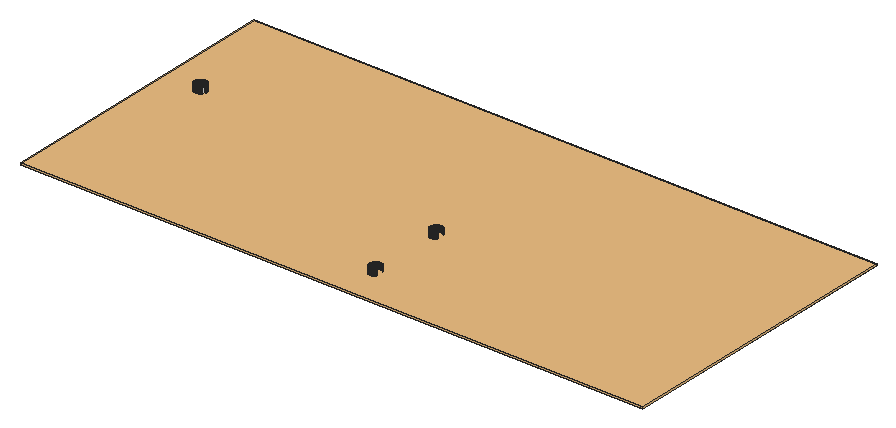
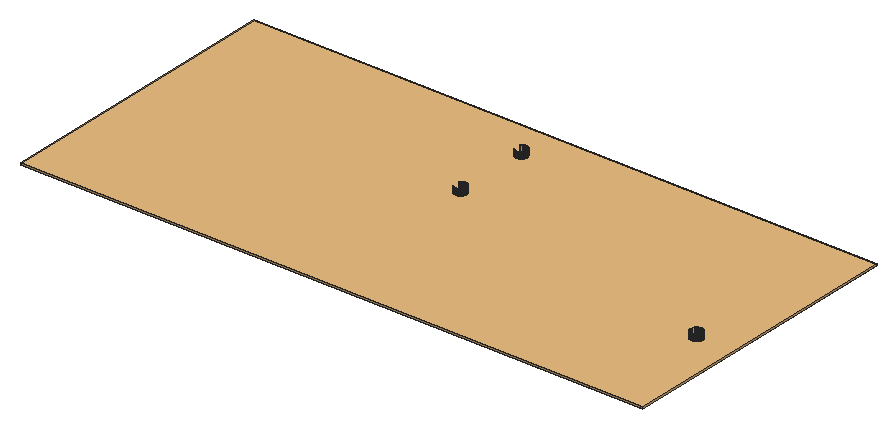
# SketchUp Ruby script. Lengths in inches.
U = 1.inch
M = Sketchup.active_model
def pt(a) = Geom::Point3d.new(a.map { |v| v * U })
def face(e, loops, mat)
  f = e.add_face(loops[0].map { |a| pt(a) })
  loops[1..].each { |l| e.add_face(l.map { |a| pt(a) }).erase! }
  f.material = f.back_material = mat if mat
  f
end
# faces: each face lists its corners as indices into pts; further lists are holes
def faces(e, pts, list, mat = nil) = list.each { |f| face(e, (f[0].is_a?(Array) ? f : [f]).map { |l| l.map { |i| pts[i] } }, mat) }
# xy, xz, yz: faces in a plane at the given z, y or x. An outline is a flat list of corners, or four numbers for a rectangle; further outlines are holes
def ring(l) = l.size == 4 ? [[l[0], l[1]], [l[2], l[1]], [l[2], l[3]], [l[0], l[3]]] : l.each_slice(2).to_a
def flat(e, list, mat, &to3) = list.each { |f| face(e, (f[0].is_a?(Array) ? f : [f]).map { |l| ring(l).map { |u, v| to3.(u, v) } }, mat) }
def xy(e, z, list, mat = nil) = flat(e, list, mat) { |x, y| [x, y, z] }
def xz(e, y, list, mat = nil) = flat(e, list, mat) { |x, z| [x, y, z] }
def yz(e, x, list, mat = nil) = flat(e, list, mat) { |y, z| [x, y, z] }
def lines(e, pts, list) = list.each { |a, b| e.add_line(pt(pts[a]), pt(pts[b])) }
# prism: a flat outline (further loops are holes) pulled along v
def prism(e, loops, v, mat = nil)
  f = face(e, loops, mat); d = Geom::Vector3d.new(v.map { |x| x * U })
  f.pushpull(f.normal.samedirection?(d) ? d.length : -d.length)
end
def box(e, o, s, mat = nil) = prism(e, [[o, [o[0] + s[0], o[1], o[2]], [o[0] + s[0], o[1] + s[1], o[2]], [o[0], o[1] + s[1], o[2]]]], [0, 0, s[2]], mat)
def at(x, y, z, deg = 0) = Geom::Transformation.translation(pt([x, y, z])) * Geom::Transformation.rotation(ORIGIN, Z_AXIS, deg.degrees)
def axes(o, x, y, z) = Geom::Transformation.new([*x, 0, *y, 0, *z, 0, *pt(o).to_a, 1])
def part(name) = M.definitions.add(name)
# library, detail: a bought-in or finely detailed component or shape, given as its bounding box
def library(name, o, s) = part(name).tap { |d| box(d.entities, o, s) }
def detail(e, o, s) = box(e.add_group.entities, o, s)
def put(e, d, t, mat = nil) = e.add_instance(d, t).tap { |i| i.material = mat if mat }
def group(e, t, mat = nil) = e.add_group.tap { |g| g.transformation = t; g.material = mat if mat }.entities
root = M.entities
M.materials.add("False Ceiling Light").color = [251, 213, 131]
c1 = library("Group\#31",[0,0,0],[264,124,0.5])
xz(root,137.5,[[159.84,116,159.92,119],[159.92,116,160,119],[160,116,160.08,119],[160.08,116,160.16,119]])
xz(root,142.5,[[159.84,116,159.92,119],[159.92,116,160,119],[160,116,160.08,119],[160.08,116,160.16,119]])
xz(root,169.5,[[159.84,116,159.92,119],[159.92,116,160,119],[160,116,160.08,119],[160.08,116,160.16,119]])
xz(root,174.5,[[159.84,116,159.92,119],[159.92,116,160,119],[160,116,160.08,119],[160.08,116,160.16,119]])
xz(root,197.5,[[37.34,116,37.42,119],[37.42,116,37.5,119],[37.5,116,37.58,119],[37.58,116,37.66,119]])
xz(root,202.5,[[37.34,116,37.42,119],[37.42,116,37.5,119],[37.5,116,37.58,119],[37.58,116,37.66,119]])
yz(root,35,[[199.84,116,199.92,119],[199.92,116,200,119],[200,116,200.08,119],[200.08,116,200.16,119]])
yz(root,40,[[200,116,200.08,119],[200.08,116,200.16,119]])
yz(root,157.5,[[139.84,116,139.92,119],[139.92,116,140,119],[140,116,140.08,119],[140.08,116,140.16,119],[171.84,116,171.92,119],
  [171.92,116,172,119],[172,116,172.08,119],[172.08,116,172.16,119]])
p = [[159.53,137.54,116],[159.45,137.56,116],[159.45,137.56,119],[159.53,137.54,119],[159.61,137.53,116],[159.61,137.53,119],
  [159.6875,137.52,116],[159.6875,137.52,119],[159.76,137.51,116],[159.76,137.51,119],[159.84,137.5,116],[159.84,137.5,119],
  [160.24,137.51,116],[160.16,137.5,116],[160.16,137.5,119],[160.24,137.51,119],[160.3125,137.52,116],[160.3125,137.52,119],
  [160.39,137.53,116],[160.39,137.53,119],[160.47,137.54,116],[160.47,137.54,119],[160.55,137.56,116],[160.55,137.56,119],
  [159.15,137.65,116],[159.08,137.68,116],[159.08,137.68,119],[159.15,137.65,119],[159.23,137.62,116],[159.23,137.62,119],
  [159.3,137.6,116],[159.3,137.6,119],[159.38,137.58,116],[159.38,137.58,119],[160.62,137.58,116],[160.62,137.58,119],
  [160.7,137.6,116],[160.7,137.6,119],[160.77,137.62,116],[160.77,137.62,119],[160.85,137.65,116],[160.85,137.65,119],
  [160.92,137.68,116],[160.92,137.68,119],[158.9375,137.74,116],[158.87,137.77,116],[158.87,137.77,119],[158.9375,137.74,119],
  [159.01,137.71,116],[159.01,137.71,119],[160.99,137.71,116],[160.99,137.71,119],[161.0625,137.74,116],[161.0625,137.74,119],
  [161.13,137.77,116],[161.13,137.77,119],[158.73,137.85,116],[158.66,137.89,116],[158.66,137.89,119],[158.73,137.85,119],
  [158.8,137.81,116],[158.8,137.81,119],[161.2,137.81,116],[161.2,137.81,119],[161.27,137.85,116],[161.27,137.85,119],
  [161.34,137.89,116],[161.34,137.89,119],[158.59,137.93,116],[158.53,137.98,116],[158.53,137.98,119],[158.59,137.93,119],
  [161.41,137.93,116],[161.41,137.93,119],[161.47,137.98,116],[161.47,137.98,119],[158.47,138.02,116],[158.41,138.07,116],
  [158.41,138.07,119],[158.47,138.02,119],[161.53,138.02,116],[161.53,138.02,119],[161.59,138.07,116],[161.59,138.07,119],
  [158.35,138.125,116],[158.29,138.18,116],[158.29,138.18,119],[158.35,138.125,119],[161.65,138.125,116],[161.65,138.125,119],
  [161.71,138.18,116],[161.71,138.18,119],[158.23,138.23,116],[158.18,138.29,116],[158.18,138.29,119],[158.23,138.23,119],
  [161.77,138.23,116],[161.77,138.23,119],[161.82,138.29,116],[161.82,138.29,119],[158.125,138.35,116],[158.07,138.41,116],
  [158.07,138.41,119],[158.125,138.35,119],[161.875,138.35,116],[161.875,138.35,119],[158.02,138.47,116],[158.02,138.47,119],
  [157.98,138.53,116],[157.93,138.59,116],[157.93,138.59,119],[157.98,138.53,119],[157.89,138.66,116],[157.89,138.66,119],
  [157.85,138.73,116],[157.81,138.8,116],[157.81,138.8,119],[157.85,138.73,119],[157.77,138.87,116],[157.77,138.87,119],
  [157.74,138.9375,116],[157.71,139.01,116],[157.71,139.01,119],[157.74,138.9375,119],[157.68,139.08,116],[157.68,139.08,119],
  [157.65,139.15,116],[157.65,139.15,119],[157.62,139.23,116],[157.6,139.3,116],[157.6,139.3,119],[157.62,139.23,119],
  [157.58,139.38,116],[157.58,139.38,119],[157.56,139.45,116],[157.56,139.45,119],[157.54,139.53,116],[157.53,139.61,116],
  [157.53,139.61,119],[157.54,139.53,119],[157.52,139.6875,116],[157.52,139.6875,119],[157.51,139.76,116],[157.51,139.76,119],
  [157.5,139.84,116],[157.5,139.84,119],[157.5,140.16,116],[157.51,140.24,116],[157.51,140.24,119],[157.5,140.16,119],
  [157.52,140.3125,116],[157.52,140.3125,119],[157.53,140.39,116],[157.53,140.39,119],[157.54,140.47,116],[157.54,140.47,119],
  [157.56,140.55,116],[157.56,140.55,119],[157.58,140.62,116],[157.58,140.62,119],[157.6,140.7,116],[157.6,140.7,119],
  [157.62,140.77,116],[157.62,140.77,119],[157.65,140.85,116],[157.65,140.85,119],[157.68,140.92,116],[157.68,140.92,119],
  [157.71,140.99,116],[157.71,140.99,119],[157.74,141.0625,116],[157.74,141.0625,119],[157.77,141.13,116],[157.77,141.13,119],
  [157.81,141.2,116],[157.81,141.2,119],[157.85,141.27,116],[157.85,141.27,119],[157.89,141.34,116],[157.89,141.34,119],
  [157.93,141.41,116],[157.93,141.41,119],[157.98,141.47,116],[157.98,141.47,119],[158.02,141.53,116],[158.02,141.53,119],
  [158.07,141.59,116],[158.07,141.59,119],[158.125,141.65,116],[158.125,141.65,119],[158.18,141.71,116],[158.18,141.71,119],
  [158.23,141.77,116],[158.23,141.77,119],[161.77,141.77,116],[161.82,141.71,116],[161.82,141.71,119],[161.77,141.77,119],
  [158.29,141.82,116],[158.29,141.82,119],[158.35,141.875,116],[158.35,141.875,119],[161.65,141.875,116],[161.71,141.82,116],
  [161.71,141.82,119],[161.65,141.875,119],[158.41,141.93,116],[158.41,141.93,119],[158.47,141.98,116],[158.47,141.98,119],
  [161.53,141.98,116],[161.59,141.93,116],[161.59,141.93,119],[161.53,141.98,119],[158.53,142.02,116],[158.53,142.02,119],
  [158.59,142.07,116],[158.59,142.07,119],[161.41,142.07,116],[161.47,142.02,116],[161.47,142.02,119],[161.41,142.07,119],
  [158.66,142.11,116],[158.66,142.11,119],[158.73,142.15,116],[158.73,142.15,119],[161.27,142.15,116],[161.34,142.11,116],
  [161.34,142.11,119],[161.27,142.15,119],[158.8,142.19,116],[158.8,142.19,119],[158.87,142.23,116],[158.87,142.23,119],
  [158.9375,142.26,116],[158.9375,142.26,119],[161.0625,142.26,116],[161.13,142.23,116],[161.13,142.23,119],[161.0625,142.26,119],
  [161.2,142.19,116],[161.2,142.19,119],[159.01,142.29,116],[159.01,142.29,119],[159.08,142.32,116],[159.08,142.32,119],
  [159.15,142.35,116],[159.15,142.35,119],[160.85,142.35,116],[160.92,142.32,116],[160.92,142.32,119],[160.85,142.35,119],
  [160.99,142.29,116],[160.99,142.29,119],[159.23,142.38,116],[159.23,142.38,119],[159.3,142.4,116],[159.3,142.4,119],
  [159.38,142.42,116],[159.38,142.42,119],[159.45,142.44,116],[159.45,142.44,119],[159.53,142.46,116],[159.53,142.46,119],
  [160.47,142.46,116],[160.55,142.44,116],[160.55,142.44,119],[160.47,142.46,119],[160.62,142.42,116],[160.62,142.42,119],
  [160.7,142.4,116],[160.7,142.4,119],[160.77,142.38,116],[160.77,142.38,119],[159.61,142.47,116],[159.61,142.47,119],
  [159.6875,142.48,116],[159.6875,142.48,119],[159.76,142.49,116],[159.76,142.49,119],[159.84,142.5,116],[159.84,142.5,119],
  [160.16,142.5,116],[160.24,142.49,116],[160.24,142.49,119],[160.16,142.5,119],[160.3125,142.48,116],[160.3125,142.48,119],
  [160.39,142.47,116],[160.39,142.47,119],[159.53,169.54,116],[159.45,169.56,116],[159.45,169.56,119],[159.53,169.54,119],
  [159.61,169.53,116],[159.61,169.53,119],[159.6875,169.52,116],[159.6875,169.52,119],[159.76,169.51,116],[159.76,169.51,119],
  [159.84,169.5,116],[159.84,169.5,119],[160.24,169.51,116],[160.16,169.5,116],[160.16,169.5,119],[160.24,169.51,119],
  [160.3125,169.52,116],[160.3125,169.52,119],[160.39,169.53,116],[160.39,169.53,119],[160.47,169.54,116],[160.47,169.54,119],
  [160.55,169.56,116],[160.55,169.56,119],[159.15,169.65,116],[159.08,169.68,116],[159.08,169.68,119],[159.15,169.65,119],
  [159.23,169.62,116],[159.23,169.62,119],[159.3,169.6,116],[159.3,169.6,119],[159.38,169.58,116],[159.38,169.58,119],
  [160.62,169.58,116],[160.62,169.58,119],[160.7,169.6,116],[160.7,169.6,119],[160.77,169.62,116],[160.77,169.62,119],
  [160.85,169.65,116],[160.85,169.65,119],[160.92,169.68,116],[160.92,169.68,119],[158.9375,169.74,116],[158.87,169.77,116],
  [158.87,169.77,119],[158.9375,169.74,119],[159.01,169.71,116],[159.01,169.71,119],[160.99,169.71,116],[160.99,169.71,119],
  [161.0625,169.74,116],[161.0625,169.74,119],[161.13,169.77,116],[161.13,169.77,119],[158.73,169.85,116],[158.66,169.89,116],
  [158.66,169.89,119],[158.73,169.85,119],[158.8,169.81,116],[158.8,169.81,119],[161.2,169.81,116],[161.2,169.81,119],
  [161.27,169.85,116],[161.27,169.85,119],[161.34,169.89,116],[161.34,169.89,119],[158.59,169.93,116],[158.53,169.98,116],
  [158.53,169.98,119],[158.59,169.93,119],[161.41,169.93,116],[161.41,169.93,119],[161.47,169.98,116],[161.47,169.98,119],
  [158.47,170.02,116],[158.41,170.07,116],[158.41,170.07,119],[158.47,170.02,119],[161.53,170.02,116],[161.53,170.02,119],
  [161.59,170.07,116],[161.59,170.07,119],[158.35,170.125,116],[158.29,170.18,116],[158.29,170.18,119],[158.35,170.125,119],
  [161.65,170.125,116],[161.65,170.125,119],[161.71,170.18,116],[161.71,170.18,119],[158.23,170.23,116],[158.18,170.29,116],
  [158.18,170.29,119],[158.23,170.23,119],[161.77,170.23,116],[161.77,170.23,119],[161.82,170.29,116],[161.82,170.29,119],
  [158.125,170.35,116],[158.07,170.41,116],[158.07,170.41,119],[158.125,170.35,119],[161.875,170.35,116],[161.875,170.35,119],
  [158.02,170.47,116],[158.02,170.47,119],[157.98,170.53,116],[157.93,170.59,116],[157.93,170.59,119],[157.98,170.53,119],
  [157.89,170.66,116],[157.89,170.66,119],[157.85,170.73,116],[157.81,170.8,116],[157.81,170.8,119],[157.85,170.73,119],
  [157.77,170.87,116],[157.77,170.87,119],[157.74,170.9375,116],[157.71,171.01,116],[157.71,171.01,119],[157.74,170.9375,119],
  [157.68,171.08,116],[157.68,171.08,119],[157.65,171.15,116],[157.65,171.15,119],[157.62,171.23,116],[157.6,171.3,116],
  [157.6,171.3,119],[157.62,171.23,119],[157.58,171.38,116],[157.58,171.38,119],[157.56,171.45,116],[157.56,171.45,119],
  [157.54,171.53,116],[157.53,171.61,116],[157.53,171.61,119],[157.54,171.53,119],[157.52,171.6875,116],[157.52,171.6875,119],
  [157.51,171.76,116],[157.51,171.76,119],[157.5,171.84,116],[157.5,171.84,119],[157.5,172.16,116],[157.51,172.24,116],
  [157.51,172.24,119],[157.5,172.16,119],[157.52,172.3125,116],[157.52,172.3125,119],[157.53,172.39,116],[157.53,172.39,119],
  [157.54,172.47,116],[157.54,172.47,119],[157.56,172.55,116],[157.56,172.55,119],[157.58,172.62,116],[157.58,172.62,119],
  [157.6,172.7,116],[157.6,172.7,119],[157.62,172.77,116],[157.62,172.77,119],[157.65,172.85,116],[157.65,172.85,119],
  [157.68,172.92,116],[157.68,172.92,119],[157.71,172.99,116],[157.71,172.99,119],[157.74,173.0625,116],[157.74,173.0625,119],
  [157.77,173.13,116],[157.77,173.13,119],[157.81,173.2,116],[157.81,173.2,119],[157.85,173.27,116],[157.85,173.27,119],
  [157.89,173.34,116],[157.89,173.34,119],[157.93,173.41,116],[157.93,173.41,119],[157.98,173.47,116],[157.98,173.47,119],
  [158.02,173.53,116],[158.02,173.53,119],[158.07,173.59,116],[158.07,173.59,119],[158.125,173.65,116],[158.125,173.65,119],
  [158.18,173.71,116],[158.18,173.71,119],[158.23,173.77,116],[158.23,173.77,119],[161.77,173.77,116],[161.82,173.71,116],
  [161.82,173.71,119],[161.77,173.77,119],[161.875,173.65,116],[161.875,173.65,119],[158.29,173.82,116],[158.29,173.82,119],
  [158.35,173.875,116],[158.35,173.875,119],[161.65,173.875,116],[161.71,173.82,116],[161.71,173.82,119],[161.65,173.875,119],
  [158.41,173.93,116],[158.41,173.93,119],[158.47,173.98,116],[158.47,173.98,119],[161.53,173.98,116],[161.59,173.93,116],
  [161.59,173.93,119],[161.53,173.98,119],[158.53,174.02,116],[158.53,174.02,119],[158.59,174.07,116],[158.59,174.07,119],
  [161.41,174.07,116],[161.47,174.02,116],[161.47,174.02,119],[161.41,174.07,119],[158.66,174.11,116],[158.66,174.11,119],
  [158.73,174.15,116],[158.73,174.15,119],[161.27,174.15,116],[161.34,174.11,116],[161.34,174.11,119],[161.27,174.15,119],
  [158.8,174.19,116],[158.8,174.19,119],[158.87,174.23,116],[158.87,174.23,119],[158.9375,174.26,116],[158.9375,174.26,119],
  [161.0625,174.26,116],[161.13,174.23,116],[161.13,174.23,119],[161.0625,174.26,119],[161.2,174.19,116],[161.2,174.19,119],
  [159.01,174.29,116],[159.01,174.29,119],[159.08,174.32,116],[159.08,174.32,119],[159.15,174.35,116],[159.15,174.35,119],
  [160.85,174.35,116],[160.92,174.32,116],[160.92,174.32,119],[160.85,174.35,119],[160.99,174.29,116],[160.99,174.29,119],
  [159.23,174.38,116],[159.23,174.38,119],[159.3,174.4,116],[159.3,174.4,119],[159.38,174.42,116],[159.38,174.42,119],
  [159.45,174.44,116],[159.45,174.44,119],[159.53,174.46,116],[159.53,174.46,119],[160.47,174.46,116],[160.55,174.44,116],
  [160.55,174.44,119],[160.47,174.46,119],[160.62,174.42,116],[160.62,174.42,119],[160.7,174.4,116],[160.7,174.4,119],
  [160.77,174.38,116],[160.77,174.38,119],[159.61,174.47,116],[159.61,174.47,119],[159.6875,174.48,116],[159.6875,174.48,119],
  [159.76,174.49,116],[159.76,174.49,119],[159.84,174.5,116],[159.84,174.5,119],[160.16,174.5,116],[160.24,174.49,116],
  [160.24,174.49,119],[160.16,174.5,119],[160.3125,174.48,116],[160.3125,174.48,119],[160.39,174.47,116],[160.39,174.47,119],
  [37.03,197.54,116],[36.95,197.56,116],[36.95,197.56,119],[37.03,197.54,119],[37.11,197.53,116],[37.11,197.53,119],
  [37.1875,197.52,116],[37.1875,197.52,119],[37.26,197.51,116],[37.26,197.51,119],[37.34,197.5,116],[37.34,197.5,119],
  [37.74,197.51,116],[37.66,197.5,116],[37.66,197.5,119],[37.74,197.51,119],[37.8125,197.52,116],[37.8125,197.52,119],
  [37.89,197.53,116],[37.89,197.53,119],[37.97,197.54,116],[37.97,197.54,119],[38.05,197.56,116],[38.05,197.56,119],
  [36.65,197.65,116],[36.58,197.68,116],[36.58,197.68,119],[36.65,197.65,119],[36.73,197.62,116],[36.73,197.62,119],
  [36.8,197.6,116],[36.8,197.6,119],[36.88,197.58,116],[36.88,197.58,119],[38.12,197.58,116],[38.12,197.58,119],
  [38.2,197.6,116],[38.2,197.6,119],[38.27,197.62,116],[38.27,197.62,119],[38.35,197.65,116],[38.35,197.65,119],
  [38.42,197.68,116],[38.42,197.68,119],[36.4375,197.74,116],[36.37,197.77,116],[36.37,197.77,119],[36.4375,197.74,119],
  [36.51,197.71,116],[36.51,197.71,119],[38.49,197.71,116],[38.49,197.71,119],[38.5625,197.74,116],[38.5625,197.74,119],
  [38.63,197.77,116],[38.63,197.77,119],[36.23,197.85,116],[36.16,197.89,116],[36.16,197.89,119],[36.23,197.85,119],
  [36.3,197.81,116],[36.3,197.81,119],[38.7,197.81,116],[38.7,197.81,119],[38.77,197.85,116],[38.77,197.85,119],
  [38.84,197.89,116],[38.84,197.89,119],[36.09,197.93,116],[36.03,197.98,116],[36.03,197.98,119],[36.09,197.93,119],
  [38.91,197.93,116],[38.91,197.93,119],[38.97,197.98,116],[38.97,197.98,119],[35.97,198.02,116],[35.91,198.07,116],
  [35.91,198.07,119],[35.97,198.02,119],[39.03,198.02,116],[39.03,198.02,119],[39.09,198.07,116],[39.09,198.07,119],
  [35.85,198.125,116],[35.79,198.18,116],[35.79,198.18,119],[35.85,198.125,119],[39.15,198.125,116],[39.15,198.125,119],
  [39.21,198.18,116],[39.21,198.18,119],[35.73,198.23,116],[35.68,198.29,116],[35.68,198.29,119],[35.73,198.23,119],
  [39.27,198.23,116],[39.27,198.23,119],[39.32,198.29,116],[39.32,198.29,119],[35.625,198.35,116],[35.57,198.41,116],
  [35.57,198.41,119],[35.625,198.35,119],[39.375,198.35,116],[39.375,198.35,119],[39.43,198.41,116],[39.43,198.41,119],
  [35.52,198.47,116],[35.52,198.47,119],[39.48,198.47,116],[39.48,198.47,119],[35.48,198.53,116],[35.43,198.59,116],
  [35.43,198.59,119],[35.48,198.53,119],[39.52,198.53,116],[39.52,198.53,119],[39.57,198.59,116],[39.57,198.59,119],
  [35.39,198.66,116],[35.39,198.66,119],[39.61,198.66,116],[39.61,198.66,119],[35.35,198.73,116],[35.31,198.8,116],
  [35.31,198.8,119],[35.35,198.73,119],[39.65,198.73,116],[39.65,198.73,119],[39.69,198.8,116],[39.69,198.8,119],
  [35.27,198.87,116],[35.27,198.87,119],[39.73,198.87,116],[39.73,198.87,119],[35.24,198.9375,116],[35.21,199.01,116],
  [35.21,199.01,119],[35.24,198.9375,119],[39.76,198.9375,116],[39.76,198.9375,119],[35.18,199.08,116],[35.18,199.08,119],
  [35.15,199.15,116],[35.15,199.15,119],[35.12,199.23,116],[35.1,199.3,116],[35.1,199.3,119],[35.12,199.23,119],
  [35.08,199.38,116],[35.08,199.38,119],[35.06,199.45,116],[35.06,199.45,119],[35.04,199.53,116],[35.03,199.61,116],
  [35.03,199.61,119],[35.04,199.53,119],[35.02,199.6875,116],[35.02,199.6875,119],[35.01,199.76,116],[35.01,199.76,119],
  [35,199.84,116],[35,199.84,119],[35,200.16,116],[35.01,200.24,116],[35.01,200.24,119],[35,200.16,119],
  [35.02,200.3125,116],[35.02,200.3125,119],[39.98,200.3125,116],[39.99,200.24,116],[39.99,200.24,119],[39.98,200.3125,119],
  [40,200.16,116],[40,200.16,119],[35.03,200.39,116],[35.03,200.39,119],[39.97,200.39,116],[39.97,200.39,119],
  [35.04,200.47,116],[35.04,200.47,119],[39.96,200.47,116],[39.96,200.47,119],[35.06,200.55,116],[35.06,200.55,119],
  [35.08,200.62,116],[35.08,200.62,119],[39.92,200.62,116],[39.94,200.55,116],[39.94,200.55,119],[39.92,200.62,119],
  [35.1,200.7,116],[35.1,200.7,119],[39.9,200.7,116],[39.9,200.7,119],[35.12,200.77,116],[35.12,200.77,119],
  [39.88,200.77,116],[39.88,200.77,119],[35.15,200.85,116],[35.15,200.85,119],[35.18,200.92,116],[35.18,200.92,119],
  [39.82,200.92,116],[39.85,200.85,116],[39.85,200.85,119],[39.82,200.92,119],[35.21,200.99,116],[35.21,200.99,119],
  [39.79,200.99,116],[39.79,200.99,119],[35.24,201.0625,116],[35.24,201.0625,119],[39.76,201.0625,116],[39.76,201.0625,119],
  [35.27,201.13,116],[35.27,201.13,119],[35.31,201.2,116],[35.31,201.2,119],[39.69,201.2,116],[39.73,201.13,116],
  [39.73,201.13,119],[39.69,201.2,119],[35.35,201.27,116],[35.35,201.27,119],[39.65,201.27,116],[39.65,201.27,119],
  [35.39,201.34,116],[35.39,201.34,119],[35.43,201.41,116],[35.43,201.41,119],[39.57,201.41,116],[39.61,201.34,116],
  [39.61,201.34,119],[39.57,201.41,119],[35.48,201.47,116],[35.48,201.47,119],[39.52,201.47,116],[39.52,201.47,119],
  [35.52,201.53,116],[35.52,201.53,119],[35.57,201.59,116],[35.57,201.59,119],[39.43,201.59,116],[39.48,201.53,116],
  [39.48,201.53,119],[39.43,201.59,119],[35.625,201.65,116],[35.625,201.65,119],[39.375,201.65,116],[39.375,201.65,119],
  [35.68,201.71,116],[35.68,201.71,119],[35.73,201.77,116],[35.73,201.77,119],[39.27,201.77,116],[39.32,201.71,116],
  [39.32,201.71,119],[39.27,201.77,119],[35.79,201.82,116],[35.79,201.82,119],[35.85,201.875,116],[35.85,201.875,119],
  [39.15,201.875,116],[39.21,201.82,116],[39.21,201.82,119],[39.15,201.875,119],[35.91,201.93,116],[35.91,201.93,119],
  [35.97,201.98,116],[35.97,201.98,119],[39.03,201.98,116],[39.09,201.93,116],[39.09,201.93,119],[39.03,201.98,119],
  [36.03,202.02,116],[36.03,202.02,119],[36.09,202.07,116],[36.09,202.07,119],[38.91,202.07,116],[38.97,202.02,116],
  [38.97,202.02,119],[38.91,202.07,119],[36.16,202.11,116],[36.16,202.11,119],[36.23,202.15,116],[36.23,202.15,119],
  [38.77,202.15,116],[38.84,202.11,116],[38.84,202.11,119],[38.77,202.15,119],[36.3,202.19,116],[36.3,202.19,119],
  [36.37,202.23,116],[36.37,202.23,119],[36.4375,202.26,116],[36.4375,202.26,119],[38.5625,202.26,116],[38.63,202.23,116],
  [38.63,202.23,119],[38.5625,202.26,119],[38.7,202.19,116],[38.7,202.19,119],[36.51,202.29,116],[36.51,202.29,119],
  [36.58,202.32,116],[36.58,202.32,119],[36.65,202.35,116],[36.65,202.35,119],[38.35,202.35,116],[38.42,202.32,116],
  [38.42,202.32,119],[38.35,202.35,119],[38.49,202.29,116],[38.49,202.29,119],[36.73,202.38,116],[36.73,202.38,119],
  [36.8,202.4,116],[36.8,202.4,119],[36.88,202.42,116],[36.88,202.42,119],[36.95,202.44,116],[36.95,202.44,119],
  [37.03,202.46,116],[37.03,202.46,119],[37.97,202.46,116],[38.05,202.44,116],[38.05,202.44,119],[37.97,202.46,119],
  [38.12,202.42,116],[38.12,202.42,119],[38.2,202.4,116],[38.2,202.4,119],[38.27,202.38,116],[38.27,202.38,119],
  [37.11,202.47,116],[37.11,202.47,119],[37.1875,202.48,116],[37.1875,202.48,119],[37.26,202.49,116],[37.26,202.49,119],
  [37.34,202.5,116],[37.34,202.5,119],[37.66,202.5,116],[37.74,202.49,116],[37.74,202.49,119],[37.66,202.5,119],
  [37.8125,202.48,116],[37.8125,202.48,119],[37.89,202.47,116],[37.89,202.47,119]]
faces(root,p,[[0,1,2,3],[4,0,3,5],[6,4,5,7],[8,6,7,9],[10,8,9,11],[12,13,14,15],[16,12,15,17],[18,16,17,19],
  [20,18,19,21],[22,20,21,23],[24,25,26,27],[28,24,27,29],[30,28,29,31],[32,30,31,33],[1,32,33,2],[34,22,23,35],
  [36,34,35,37],[38,36,37,39],[40,38,39,41],[42,40,41,43],[44,45,46,47],[48,44,47,49],[25,48,49,26],[50,42,43,51],
  [52,50,51,53],[54,52,53,55],[56,57,58,59],[60,56,59,61],[45,60,61,46],[62,54,55,63],[64,62,63,65],[66,64,65,67],
  [68,69,70,71],[57,68,71,58],[72,66,67,73],[74,72,73,75],[76,77,78,79],[69,76,79,70],[80,74,75,81],[82,80,81,83],
  [84,85,86,87],[77,84,87,78],[88,82,83,89],[90,88,89,91],[92,93,94,95],[85,92,95,86],[96,90,91,97],[98,96,97,99],
  [100,101,102,103],[93,100,103,94],[104,98,99,105],[101,106,107,102],[108,109,110,111],[106,108,111,107],[109,112,113,110],[114,115,116,117],
  [112,114,117,113],[115,118,119,116],[120,121,122,123],[118,120,123,119],[121,124,125,122],[124,126,127,125],[128,129,130,131],[126,128,131,127],
  [129,132,133,130],[132,134,135,133],[136,137,138,139],[134,136,139,135],[137,140,141,138],[140,142,143,141],[142,144,145,143],[146,147,148,149],
  [147,150,151,148],[150,152,153,151],[152,154,155,153],[154,156,157,155],[156,158,159,157],[158,160,161,159],[160,162,163,161],[162,164,165,163],
  [164,166,167,165],[166,168,169,167],[168,170,171,169],[170,172,173,171],[172,174,175,173],[174,176,177,175],[176,178,179,177],[178,180,181,179],
  [180,182,183,181],[182,184,185,183],[184,186,187,185],[186,188,189,187],[188,190,191,189],[190,192,193,191],[194,195,196,197],[192,198,199,193],
  [198,200,201,199],[202,203,204,205],[203,194,197,204],[200,206,207,201],[206,208,209,207],[210,211,212,213],[211,202,205,212],[208,214,215,209],
  [214,216,217,215],[218,219,220,221],[219,210,213,220],[216,222,223,217],[222,224,225,223],[226,227,228,229],[227,218,221,228],[224,230,231,225],
  [230,232,233,231],[232,234,235,233],[236,237,238,239],[237,240,241,238],[240,226,229,241],[234,242,243,235],[242,244,245,243],[244,246,247,245],
  [248,249,250,251],[249,252,253,250],[252,236,239,253],[246,254,255,247],[254,256,257,255],[256,258,259,257],[258,260,261,259],[260,262,263,261],
  [264,265,266,267],[265,268,269,266],[268,270,271,269],[270,272,273,271],[272,248,251,273],[262,274,275,263],[274,276,277,275],[276,278,279,277],
  [278,280,281,279],[282,283,284,285],[283,286,287,284],[286,288,289,287],[288,264,267,289],[290,291,292,293],[294,290,293,295],[296,294,295,297],
  [298,296,297,299],[300,298,299,301],[302,303,304,305],[306,302,305,307],[308,306,307,309],[310,308,309,311],[312,310,311,313],[314,315,316,317],
  [318,314,317,319],[320,318,319,321],[322,320,321,323],[291,322,323,292],[324,312,313,325],[326,324,325,327],[328,326,327,329],[330,328,329,331],
  [332,330,331,333],[334,335,336,337],[338,334,337,339],[315,338,339,316],[340,332,333,341],[342,340,341,343],[344,342,343,345],[346,347,348,349],
  [350,346,349,351],[335,350,351,336],[352,344,345,353],[354,352,353,355],[356,354,355,357],[358,359,360,361],[347,358,361,348],[362,356,357,363],
  [364,362,363,365],[366,367,368,369],[359,366,369,360],[370,364,365,371],[372,370,371,373],[374,375,376,377],[367,374,377,368],[378,372,373,379],
  [380,378,379,381],[382,383,384,385],[375,382,385,376],[386,380,381,387],[388,386,387,389],[390,391,392,393],[383,390,393,384],[394,388,389,395],
  [391,396,397,392],[398,399,400,401],[396,398,401,397],[399,402,403,400],[404,405,406,407],[402,404,407,403],[405,408,409,406],[410,411,412,413],
  [408,410,413,409],[411,414,415,412],[414,416,417,415],[418,419,420,421],[416,418,421,417],[419,422,423,420],[422,424,425,423],[426,427,428,429],
  [424,426,429,425],[427,430,431,428],[430,432,433,431],[432,434,435,433],[436,437,438,439],[437,440,441,438],[440,442,443,441],[442,444,445,443],
  [444,446,447,445],[446,448,449,447],[448,450,451,449],[450,452,453,451],[452,454,455,453],[454,456,457,455],[456,458,459,457],[458,460,461,459],
  [460,462,463,461],[462,464,465,463],[464,466,467,465],[466,468,469,467],[468,470,471,469],[470,472,473,471],[472,474,475,473],[474,476,477,475],
  [476,478,479,477],[478,480,481,479],[480,482,483,481],[484,485,486,487],[485,488,489,486],[482,490,491,483],[490,492,493,491],[494,495,496,497],
  [495,484,487,496],[492,498,499,493],[498,500,501,499],[502,503,504,505],[503,494,497,504],[500,506,507,501],[506,508,509,507],[510,511,512,513],
  [511,502,505,512],[508,514,515,509],[514,516,517,515],[518,519,520,521],[519,510,513,520],[516,522,523,517],[522,524,525,523],[524,526,527,525],
  [528,529,530,531],[529,532,533,530],[532,518,521,533],[526,534,535,527],[534,536,537,535],[536,538,539,537],[540,541,542,543],[541,544,545,542],
  [544,528,531,545],[538,546,547,539],[546,548,549,547],[548,550,551,549],[550,552,553,551],[552,554,555,553],[556,557,558,559],[557,560,561,558],
  [560,562,563,561],[562,564,565,563],[564,540,543,565],[554,566,567,555],[566,568,569,567],[568,570,571,569],[570,572,573,571],[574,575,576,577],
  [575,578,579,576],[578,580,581,579],[580,556,559,581],[582,583,584,585],[586,582,585,587],[588,586,587,589],[590,588,589,591],[592,590,591,593],
  [594,595,596,597],[598,594,597,599],[600,598,599,601],[602,600,601,603],[604,602,603,605],[606,607,608,609],[610,606,609,611],[612,610,611,613],
  [614,612,613,615],[583,614,615,584],[616,604,605,617],[618,616,617,619],[620,618,619,621],[622,620,621,623],[624,622,623,625],[626,627,628,629],
  [630,626,629,631],[607,630,631,608],[632,624,625,633],[634,632,633,635],[636,634,635,637],[638,639,640,641],[642,638,641,643],[627,642,643,628],
  [644,636,637,645],[646,644,645,647],[648,646,647,649],[650,651,652,653],[639,650,653,640],[654,648,649,655],[656,654,655,657],[658,659,660,661],
  [651,658,661,652],[662,656,657,663],[664,662,663,665],[666,667,668,669],[659,666,669,660],[670,664,665,671],[672,670,671,673],[674,675,676,677],
  [667,674,677,668],[678,672,673,679],[680,678,679,681],[682,683,684,685],[675,682,685,676],[686,680,681,687],[688,686,687,689],[683,690,691,684],
  [692,688,689,693],[694,695,696,697],[690,694,697,691],[698,692,693,699],[700,698,699,701],[695,702,703,696],[704,700,701,705],[706,707,708,709],
  [702,706,709,703],[710,704,705,711],[712,710,711,713],[707,714,715,708],[716,712,713,717],[718,719,720,721],[714,718,721,715],[722,716,717,723],
  [719,724,725,720],[724,726,727,725],[728,729,730,731],[726,728,731,727],[729,732,733,730],[732,734,735,733],[736,737,738,739],[734,736,739,735],
  [737,740,741,738],[740,742,743,741],[742,744,745,743],[746,747,748,749],[747,750,751,748],[752,753,754,755],[753,756,757,754],[750,758,759,751],
  [760,752,755,761],[758,762,763,759],[764,760,761,765],[762,766,767,763],[766,768,769,767],[770,771,772,773],[771,764,765,772],[768,774,775,769],
  [776,770,773,777],[774,778,779,775],[780,776,777,781],[778,782,783,779],[782,784,785,783],[786,787,788,789],[787,780,781,788],[784,790,791,785],
  [792,786,789,793],[790,794,795,791],[796,792,793,797],[794,798,799,795],[798,800,801,799],[802,803,804,805],[803,796,797,804],[800,806,807,801],
  [808,802,805,809],[806,810,811,807],[810,812,813,811],[814,815,816,817],[815,808,809,816],[812,818,819,813],[820,814,817,821],[818,822,823,819],
  [822,824,825,823],[826,827,828,829],[827,820,821,828],[824,830,831,825],[832,826,829,833],[830,834,835,831],[834,836,837,835],[838,839,840,841],
  [839,832,833,840],[836,842,843,837],[842,844,845,843],[846,847,848,849],[847,838,841,848],[844,850,851,845],[850,852,853,851],[854,855,856,857],
  [855,846,849,856],[852,858,859,853],[858,860,861,859],[862,863,864,865],[863,854,857,864],[860,866,867,861],[866,868,869,867],[870,871,872,873],
  [871,862,865,872],[868,874,875,869],[874,876,877,875],[876,878,879,877],[880,881,882,883],[881,884,885,882],[884,870,873,885],[878,886,887,879],
  [886,888,889,887],[888,890,891,889],[892,893,894,895],[893,896,897,894],[896,880,883,897],[890,898,899,891],[898,900,901,899],[900,902,903,901],
  [902,904,905,903],[904,906,907,905],[908,909,910,911],[909,912,913,910],[912,914,915,913],[914,916,917,915],[916,892,895,917],[906,918,919,907],
  [918,920,921,919],[920,922,923,921],[922,924,925,923],[926,927,928,929],[927,930,931,928],[930,932,933,931],[932,908,911,933]])
put(root,c1,at(22,124,116),"False Ceiling Light")
